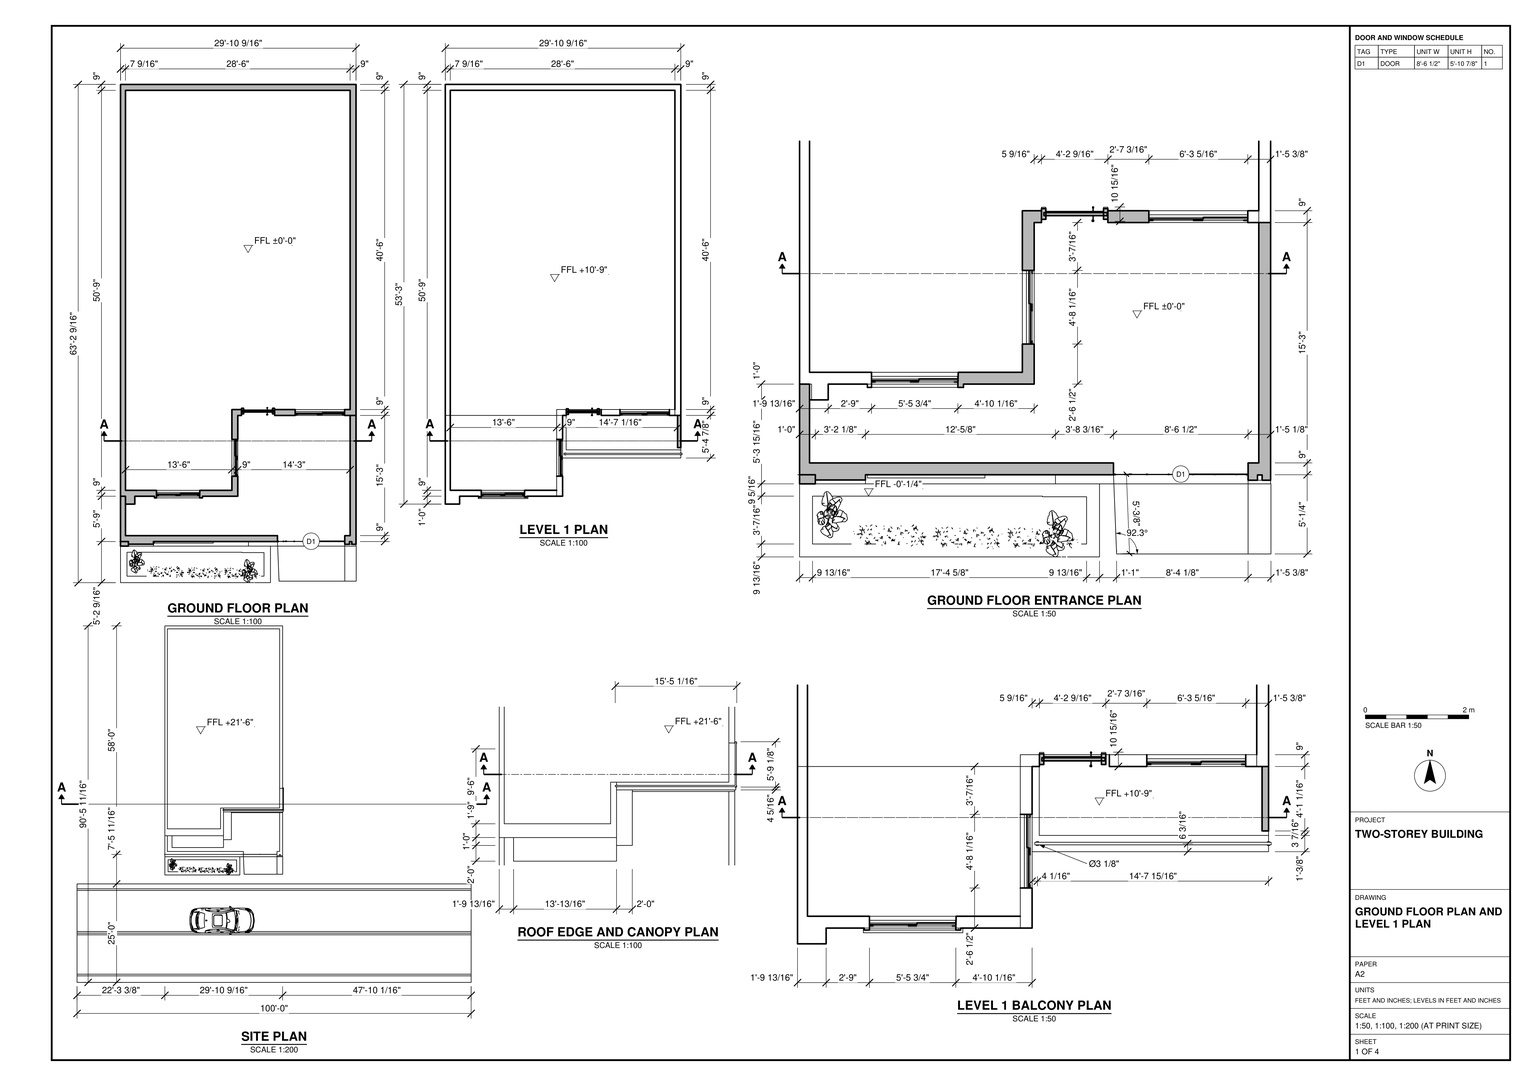
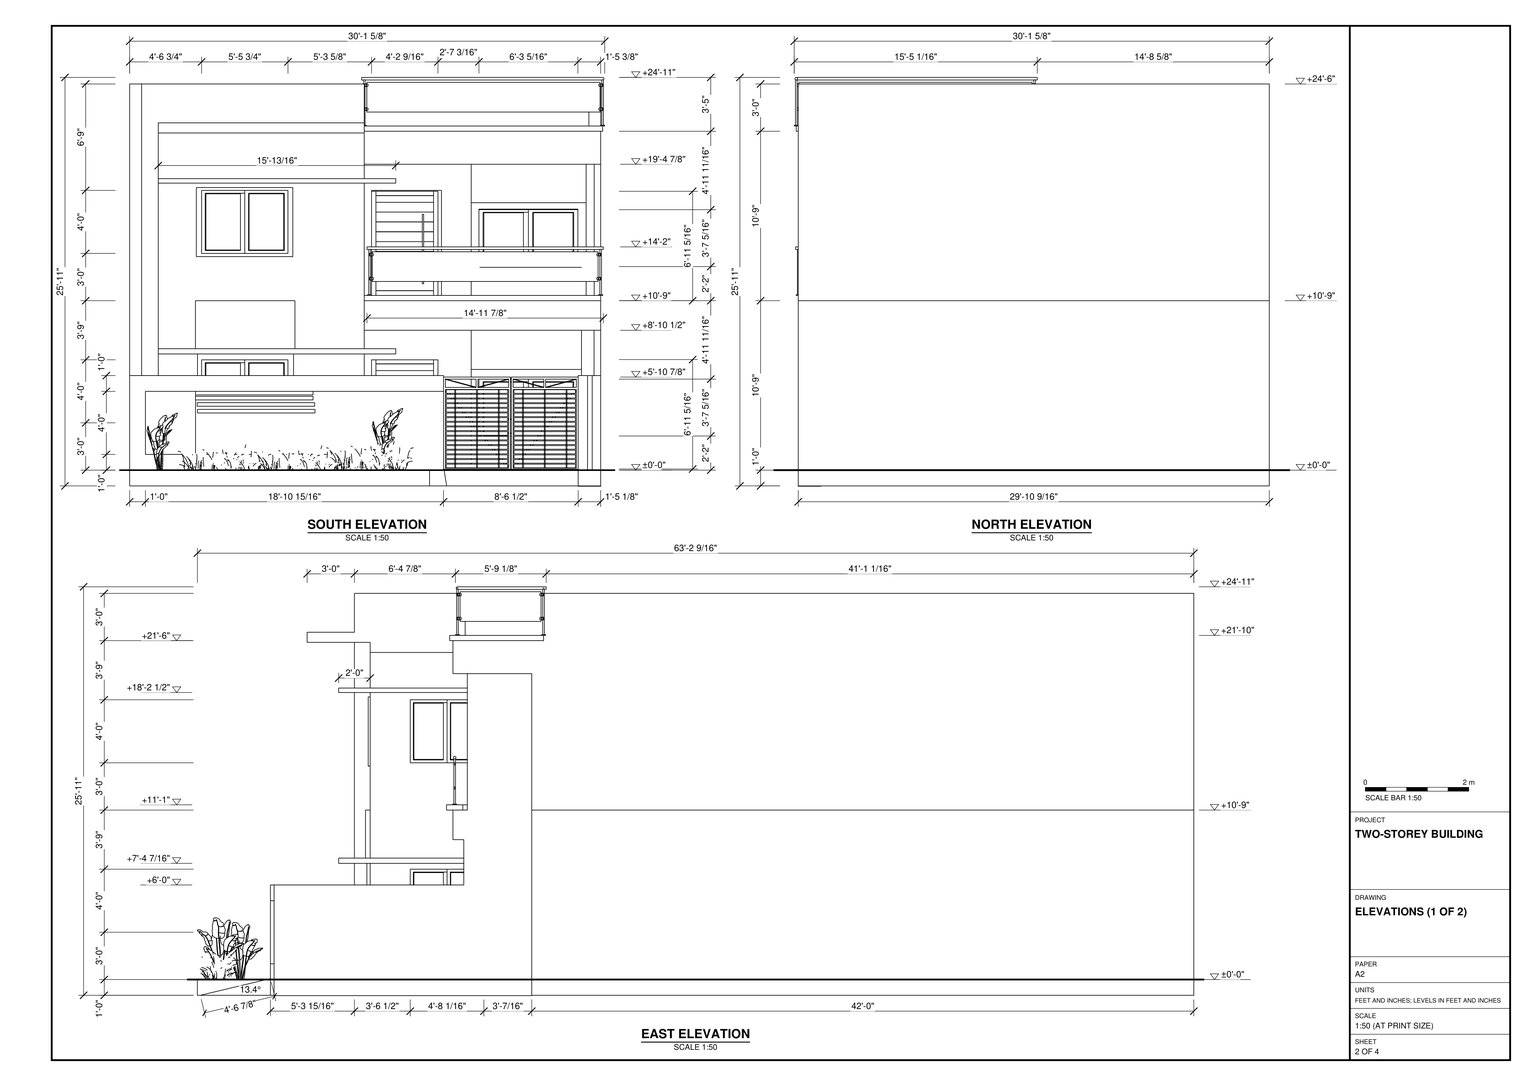
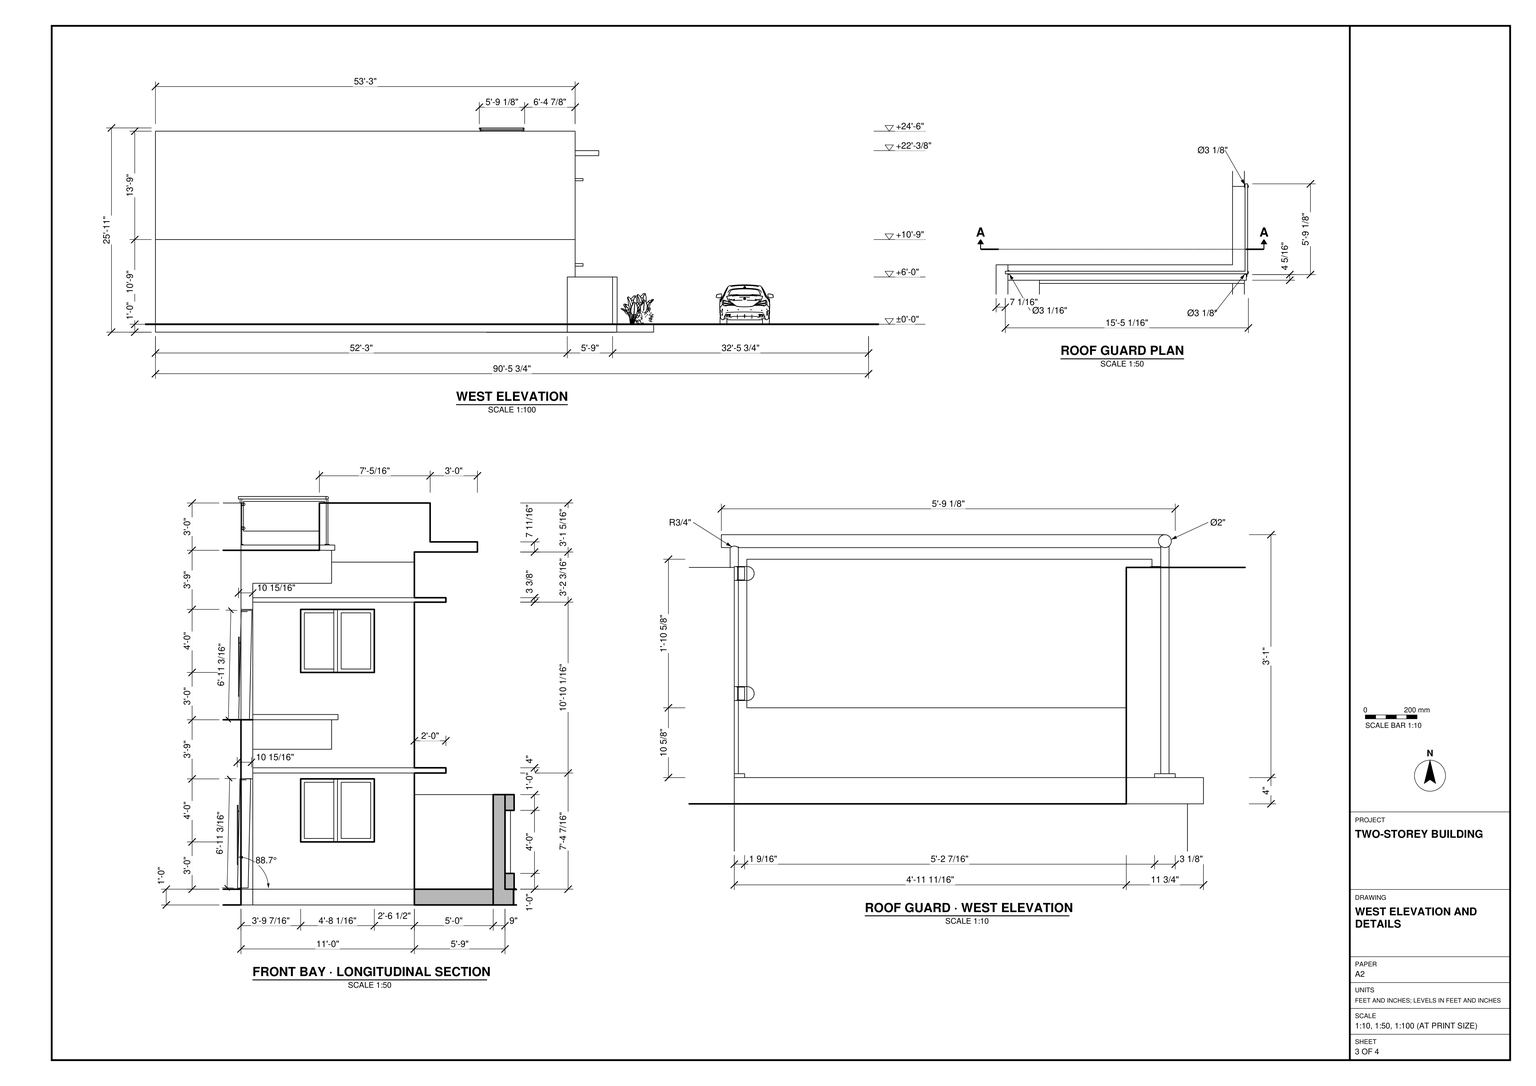
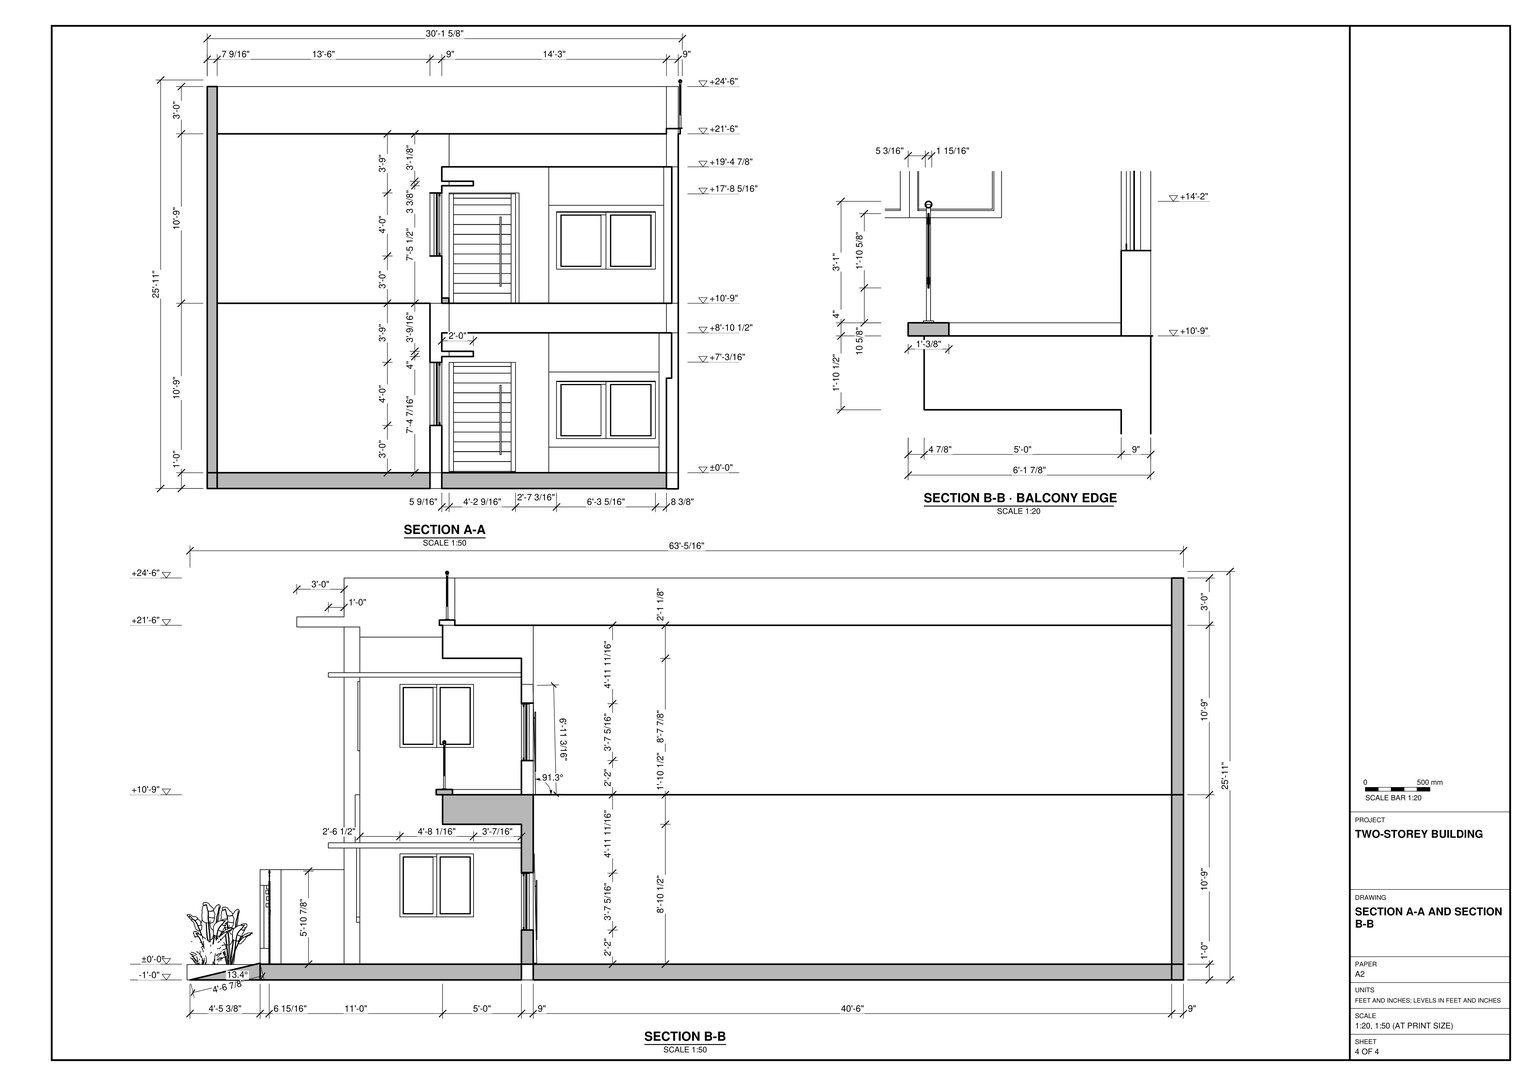
Build the two-storey building and its street frontage in SketchUp from task_files/diagram_01.pdf. Work in feet and inches. Including the site, the model shall measure 100'-0" along X, 90'-5 11/16" along Y and 25'-11 1/4" along Z. Set the ground floor at ±0'-0" and the upper floor at +10'-9".

Use the floor plans to lay out the long side walls, straight rear wall and stepped south wall. Follow the wall thicknesses shown, including the 7 9/16" west wall and 9" east wall of the main block. Model the floor slabs, flat roof and parapets. At the front, use the entrance and balcony plans to place the doors and windows on the correct faces of the stepped wall. Match the projecting canopies at both storeys and the balcony slab and guard on the recessed side. Use the roof guard detail for the posts, panels and top rail where the guard turns the roof corner.

Include the front boundary wall, slatted double gate and planting bed. Place the street across the frontage with the car positioned as in the site plan. Decor and loose items, including the plants and car, may be any suitable library components. Keep shell elements such as walls, slabs and roof, and each furniture or joinery piece, in separate groups or components; use components for repeated parts. Save one SketchUp model as output_files/two_storey_building_stepped_frontage_and_street.skp.

# SketchUp Ruby script. Lengths in inches.
U = 1.inch
M = Sketchup.active_model
def pt(a) = Geom::Point3d.new(a.map { |v| v * U })
def face(e, loops, mat)
  f = e.add_face(loops[0].map { |a| pt(a) })
  loops[1..].each { |l| e.add_face(l.map { |a| pt(a) }).erase! }
  f.material = f.back_material = mat if mat
  f
end
# faces: each face lists its corners as indices into pts; further lists are holes
def faces(e, pts, list, mat = nil) = list.each { |f| face(e, (f[0].is_a?(Array) ? f : [f]).map { |l| l.map { |i| pts[i] } }, mat) }
# xy, xz, yz: faces in a plane at the given z, y or x. An outline is a flat list of corners, or four numbers for a rectangle; further outlines are holes
def ring(l) = l.size == 4 ? [[l[0], l[1]], [l[2], l[1]], [l[2], l[3]], [l[0], l[3]]] : l.each_slice(2).to_a
def flat(e, list, mat, &to3) = list.each { |f| face(e, (f[0].is_a?(Array) ? f : [f]).map { |l| ring(l).map { |u, v| to3.(u, v) } }, mat) }
def xy(e, z, list, mat = nil) = flat(e, list, mat) { |x, y| [x, y, z] }
def xz(e, y, list, mat = nil) = flat(e, list, mat) { |x, z| [x, y, z] }
def yz(e, x, list, mat = nil) = flat(e, list, mat) { |y, z| [x, y, z] }
def lines(e, pts, list) = list.each { |a, b| e.add_line(pt(pts[a]), pt(pts[b])) }
# prism: a flat outline (further loops are holes) pulled along v
def prism(e, loops, v, mat = nil)
  f = face(e, loops, mat); d = Geom::Vector3d.new(v.map { |x| x * U })
  f.pushpull(f.normal.samedirection?(d) ? d.length : -d.length)
end
def box(e, o, s, mat = nil) = prism(e, [[o, [o[0] + s[0], o[1], o[2]], [o[0] + s[0], o[1] + s[1], o[2]], [o[0], o[1] + s[1], o[2]]]], [0, 0, s[2]], mat)
def at(x, y, z, deg = 0) = Geom::Transformation.translation(pt([x, y, z])) * Geom::Transformation.rotation(ORIGIN, Z_AXIS, deg.degrees)
def axes(o, x, y, z) = Geom::Transformation.new([*x, 0, *y, 0, *z, 0, *pt(o).to_a, 1])
def part(name) = M.definitions.add(name)
# library, detail: a bought-in or finely detailed component or shape, given as its bounding box
def library(name, o, s) = part(name).tap { |d| box(d.entities, o, s) }
def detail(e, o, s) = box(e.add_group.entities, o, s)
def put(e, d, t, mat = nil) = e.add_instance(d, t).tap { |i| i.material = mat if mat }
def group(e, t, mat = nil) = e.add_group.tap { |g| g.transformation = t; g.material = mat if mat }.entities
root = M.entities
M.materials.add("[Asphalt_New]").color = [67, 60, 62]
M.materials.add("[Color M00]").color = [255, 255, 255]
M.materials.add("[Granite Dark Gray]").color = [69, 68, 68]
M.materials.add("[Metal Seamed]").color = [118, 119, 115]
M.materials.add("[Stone Brushed Khaki]").color = [226, 197, 133]
M.materials.add("[Stone Vein Gray]").color = [166, 165, 165]
M.materials.add("[Translucent Glass Blue]").color = [100, 149, 237]
M.materials["[Translucent Glass Blue]"].alpha = 0.5
M.materials.add("[Wood Cherry Original]").color = [68, 39, 18]
M.materials.add("[Wood Cherry Original]1").color = [152, 86, 42]
M.materials.add("[Wood Floor Light]").color = [140, 99, 62]
M.materials.add("white").color = [255, 255, 255]
c1 = part("Janela aluminio")
xy(c1.entities,0,[[0,0,47.24,1.57],[23.62,1.57,47.24,2.76],[0,2.76,25.98,3.9375],[0,3.9375,47.24,5.91]])
xy(c1.entities,43.31,[[0,0,47.24,1.57],[23.62,1.57,47.24,2.76],[0,2.76,0,5.91,47.24,5.91,47.24,3.9375,25.98,3.9375,25.98,2.76],[25.98,2.76,47.24,3.9375]])
xz(c1.entities,1.57,[[0,0,23.62,0,23.62,41.34,21.26,41.34,21.26,1.97,1.97,1.97,1.97,41.34,23.62,41.34,23.62,43.31,0,43.31],[[23.62,0,47.24,43.31],[25.7,1.97,45.28,41.34]]])
xz(c1.entities,2.76,[[[0,0,23.62,43.31],[2.36,2.36,21.26,40.94]],[23.62,0,25.98,43.31]])
xz(c1.entities,2.76,[[2.36,2.36,21.26,40.94]],"[Translucent Glass Blue]")
xz(c1.entities,3.9375,[[25.98,0,25.98,2.36,44.88,2.36,44.88,40.94,25.98,40.94,25.98,43.31,47.24,43.31,47.24,0]])
xz(c1.entities,3.9375,[[25.98,2.36,44.88,40.94]],"[Translucent Glass Blue]")
yz(c1.entities,0,[[0,0,1.57,43.31],[2.76,0,5.91,43.31]])
yz(c1.entities,23.62,[[1.57,0,2.76,43.31]])
yz(c1.entities,25.98,[[2.76,0,3.9375,43.31]])
yz(c1.entities,47.24,[[0,0,1.57,43.31],[1.57,0,2.76,43.31],[3.9375,0,5.91,43.31]])
c2 = part("Agrupar\#4")
xy(c2.entities,0,[[0,0,60.82,4.875]],"[Wood Floor Light]")
c3 = part("Agrupar\#7")
box(c3.entities,[0,0,0.25],[0.65,5.875,0.35])
c4 = part("Agrupar\#15")
prism(c4.entities,[[[0,0.625,0],[0.65,0.625,0],[0.65,0,0],[0,0,0]]],[0,0.02,45.16])
c5 = part("Agrupar\#14")
put(c5.entities,c3,at(0,0.65,6.88))
put(c5.entities,c4,at(0,0,0))
put(c5.entities,c3,at(0,0.65,40.25))
c6 = part("Agrupar\#6")
prism(c6.entities,[[[-0.5,0.62,-4.9375],[0.77,0.62,-4.9375],[0.77,-0.19,-4.9375],[-0.5,-0.19,-4.9375]]],[0,0.03,52.91])
c7 = part("Agrupar\#8")
put(c7.entities,c3,at(0,0.65,6.88))
put(c7.entities,c6,at(0,0,0))
put(c7.entities,c3,at(0,0.65,40.25))
c8 = part("Agrupar\#2")
prism(c8.entities,[[[0,2.67,0.04],[55.46,2.67,0.04],[55.46,0.04,0],[0,0.04,0]]],[0,-0.04,3.23],"[Wood Cherry Original]")
c9 = part("Agrupar\#10")
prism(c9.entities,[[[0,3.76,0.04],[4.23,3.76,0.04],[4.23,1.14,0],[0,1.14,0]]],[0,-1.14,83.14],"[Wood Cherry Original]")
c10 = part("Agrupar\#1")
prism(c10.entities,[[[0,3.76,0.04],[4.23,3.76,0.04],[4.23,1.14,0],[0,1.14,0]]],[0,-1.14,83.14],"[Wood Cherry Original]")
c11 = part("Agrupar\#3")
put(c11.entities,c8,at(4.23,0,79.91))
put(c11.entities,c9,at(59.6875,0,0))
put(c11.entities,c10,at(0,0,0))
c12 = part("Agrupar\#5")
put(c12.entities,c11,axes([0,-1.34,0.11],[1,0,0],[0,3.10443,-0.05961],[0,0.0192,0.99982]))
c13 = part("Agrupar\#9")
put(c13.entities,c5,axes([49.36,10.72,17.77],[1,0,0],[0,-1,0],[0,0,1]))
put(c13.entities,c7,at(49.36,0,17.76))
put(c13.entities,c12,at(0,0.21,0.01))
c14 = part("Agrupar\#11")
box(c14.entities,[0,0,0],[60.82,4.875,7.44],"[Wood Floor Light]")
c15 = part("Agrupar\#12")
put(c15.entities,c14,at(0,0,67.34))
put(c15.entities,c14,at(0,0,44.83))
put(c15.entities,c14,at(0,0,59.9))
put(c15.entities,c14,at(0,0,74.78))
put(c15.entities,c14,at(0,0,52.37))
put(c15.entities,c14,at(0,0,7.53))
put(c15.entities,c14,at(0,0,0))
put(c15.entities,c14,at(0,0,29.95))
put(c15.entities,c14,at(0,0,15.07))
put(c15.entities,c14,at(0,0,22.51))
put(c15.entities,c14,at(0,0,37.39))
c16 = part("Agrupar\#13")
put(c16.entities,c13,at(0,0,0.0625))
put(c16.entities,c15,axes([2.375,5.17,0.15],[1,0,0],[0,0.48232,0.01095],[0,-0.02269,0.99974]))
c17 = part("PORTA PIVOTANDE ENVERNIZADA LUXURY")
p = [[59.6875,-1.28,79.91],[59.6875,-3.1,79.89],[4.23,-1.28,79.91],[4.23,-3.1,79.89]]
lines(c17.entities,p,[[0,1],[2,3]])
put(c17.entities,c2,at(0.13,-2.89,82.23))
put(c17.entities,c16,at(0,-6.8,-0.11))
c18 = library("Merbau Gate Metal Frame",[0,0,0],[4.48,115.59,70.87])
c19 = library("Banana Leaf Plant",[-4.48,-0.74,0.58],[37.34,48.6,74.1])
c20 = part("Untitled")
xy(c20.entities,0,[[140,0,145,1200],[150,0,155,1200]])
xy(c20.entities,0,[[0,0,15,1200],[20,0,140,1200],[145,0,150,1200],[155,0,275,1200],[280,0,300,1200]],"[Asphalt_New]")
xy(c20.entities,0,[[15,0,20,1200],[275,0,280,1200]],"white")
c21 = library("mercy",[0,0.0625,0.17],[86.93,197.26,61.05])
c22 = library("Group\#2",[0,0,0],[179.875,3.15,36.98])
c23 = library("Group\#3",[0,0,0],[185.04,69.11,36.98])
c24 = library("Group16",[-203.48,36.63,23.35],[29.68,67.31,27.29])
xy(root,-12.25,[[608.82,385.54,608.82,398.71,616.96,398.71,616.96,581.71,625.96,581.71,625.96,385.54]])
xy(root,-12,[[[267.38,327.15,267.38,383.28,462.18,383.28,462.18,382.78,495.69,382.78,495.69,327.15],[277.22,336.99,485.86,336.99,485.86,372.9375,452.34,372.9375,452.34,373.4375,277.22,373.4375]],[508.72,329.4,506.62,382.78,508.72,382.78],[508.72,329.4,608.82,382.78],[277.22,336.99,277.22,373.4375,452.34,373.4375,452.34,372.9375,485.86,372.9375,485.86,336.99],[506.62,382.78,506.34,389.71,506.34,398.71,274.96,398.71,274.96,458.71,276.5,458.71,276.5,446.71,289.17,446.71,289.17,458.71,445.96,458.71,445.96,581.71,451.52,581.71,451.52,590.71,436.96,590.71,436.96,467.71,274.96,467.71,274.96,1076.71,616.96,1076.71,616.96,590.71,502.08,590.71,502.08,581.71,616.96,581.71,616.96,398.71,608.82,398.71,608.82,382.78],
  [462.18,382.78,495.69,383.28],[495.69,382.78,495.69,383.28,462.18,383.28,462.18,389.71,506.34,389.71,506.62,382.78],[608.82,382.78,625.96,385.54],[267.38,383.28,267.38,458.71,274.96,458.71,274.96,398.71,506.34,398.71,506.34,389.71,462.18,389.71,462.18,383.28],[276.5,446.71,276.5,458.71,267.38,458.71,267.38,1085.71,625.96,1085.71,625.96,581.71,616.96,581.71,616.96,1076.71,274.96,1076.71,274.96,467.71,436.96,467.71,436.96,458.71,289.17,458.71,289.17,446.71]])
xy(root,-0.25,[[[267.38,327.15,495.69,327.15,495.69,382.78,462.18,382.78,462.18,383.28,267.38,383.28],[277.22,336.99,277.22,373.4375,452.34,373.4375,452.34,372.9375,485.86,372.9375,485.86,336.99]]])
xy(root,0,[[267.38,382.78,462.18,383.28],[506.62,382.78,608.82,382.78,608.82,398.71,616.96,398.71,616.96,581.71,502.08,581.71,502.08,590.71,616.96,590.71,616.96,1076.71,274.96,1076.71,274.96,467.71,436.96,467.71,436.96,590.71,451.52,590.71,451.52,581.71,445.96,581.71,445.96,458.71,289.17,458.71,289.17,446.71,274.96,446.71,274.96,398.71,506.34,398.71,506.34,389.71],[462.18,382.78,506.62,382.78,506.34,389.71,462.18,389.71],[608.82,382.78,625.96,385.54],[267.38,383.28,462.18,389.71],
  [615.96,385.54,619.5,389.54],[276.5,446.71,289.17,446.71,289.17,458.71,436.96,458.71,436.96,467.71,274.96,467.71,274.96,1076.71,616.96,1076.71,616.96,581.71,625.96,581.71,625.96,1085.71,267.38,1085.71,267.38,458.71,276.5,458.71],[274.96,446.71,276.5,458.71],[502.08,581.71,616.96,590.71]])
xy(root,12,[[279.38,382.78,317.53,385.71],[317.53,382.78,462.18,389.71],[279.38,385.71,317.53,389.71]])
xy(root,25.99,[[533.27,581.71,608.58,590.71]])
xy(root,31.89,[[319.02,456.21,392.14,458.71]])
xy(root,36,[[322.14,456.21,387.89,456.21,387.89,458.71,388.14,467.71,322.14,467.71],[436.96,489.21,445.96,545.28]])
xy(root,43.52,[[319.03,387.28,408.47,389.71],[319.03,389.71,408.47,391.71]])
xy(root,46.25,[[319.03,387.28,408.47,389.71]])
xy(root,48.65,[[318.8,387.71,408.24,389.71],[318.8,389.71,408.24,391.71]])
xy(root,51.38,[[318.8,387.71,408.24,389.71]])
xy(root,53.47,[[317.53,387.11,406.97,389.11]])
xy(root,57.27,[[317.53,387.71,406.97,389.71]])
xy(root,60,[[279.38,382.78,317.53,385.71],[317.53,382.78,317.53,387.71,406.97,387.71,406.97,389.71,494.34,389.71,494.34,382.78],[494.34,382.78,506.34,389.71],[279.38,385.71,317.53,389.71],[317.53,387.71,406.97,389.71]])
xy(root,69.74,[[533.27,581.71,608.58,590.71]])
xy(root,72,[[267.38,382.78,506.34,389.71],[608.82,385.54,615.96,385.54,615.96,389.54,619.5,389.54,619.5,385.54,625.96,385.54,625.96,529.96,620.89,529.96,620.89,581.71,616.96,581.71,616.96,398.71,608.82,398.71],[267.38,389.71,506.34,389.71,506.34,398.71,274.96,398.71,274.96,446.71,267.38,446.71],[267.38,446.71,274.96,458.71]])
xy(root,84,[[322.14,456.21,322.14,467.71,388.14,467.71,387.89,458.71,387.89,456.21],[387.89,458.71,388.14,467.71,388.14,458.71],[436.96,489.21,445.96,545.28],[451.52,581.71,502.08,590.71]])
xy(root,88.45,[[289.17,434.71,289.17,458.71,319.02,458.71,319.02,456.21,392.14,456.21,392.14,458.71,445.96,458.71,445.96,581.71,469.96,581.71,469.96,434.71],[322.14,456.21,388.14,458.71]])
xy(root,92.4375,[[289.17,434.71,469.96,434.71,469.96,581.71,445.96,581.71,445.96,458.71,393.21,458.71,393.21,455.15,317.46,455.15,317.46,458.71,289.17,458.71],[317.46,455.15,393.21,458.71]])
xy(root,106.5,[[620.89,521.71,625.96,529.96]])
xy(root,106.5,[[445.96,521.71,620.89,581.71]],"[Metal Seamed]")
xy(root,129,[[317.46,455.15,393.21,458.71],[274.96,467.71,436.96,581.71],[445.96,516.84,625.96,521.71],[445.96,521.71,625.96,521.71,625.96,529.24,451.375,529.24,451.375,581.71,445.96,581.71],[451.375,529.24,625.96,529.24,625.96,532.65,621.02,532.65,621.02,581.71,504.76,581.71,504.76,590.71,451.52,590.71,451.52,581.71,451.375,581.71],
  [267.38,581.71,274.96,581.71,274.96,1076.71,616.96,1076.71,616.96,581.71,625.96,581.71,625.96,1085.71,267.38,1085.71],[274.96,581.71,436.96,581.71,436.96,590.71,616.96,590.71,616.96,1076.71,274.96,1076.71],[436.96,581.71,451.52,590.71],[504.76,581.71,616.96,590.71]])
xy(root,133,[[445.96,516.84,625.96,516.84,625.96,529.24,451.375,529.24,451.375,581.71,445.96,581.71]])
xy(root,154.99,[[533.27,581.71,608.58,590.71]])
xy(root,162.5625,[[318.14,457.21,322.14,458.71],[322.14,457.21,390.14,458.71]])
xy(root,165,[[322.14,457.21,387.89,457.21,387.89,458.71,388.14,467.71,322.14,467.71],[436.96,489.21,445.96,545.28]])
xy(root,198.74,[[533.27,581.71,608.58,590.71]])
xy(root,213,[[322.14,457.21,322.14,467.71,388.14,467.71,387.89,458.71,387.89,457.21],[387.89,458.71,388.14,467.71,388.14,458.71],[436.96,489.21,445.96,545.28],[451.52,581.71,504.76,590.71]])
xy(root,215.15,[[318.14,457.21,322.14,458.71],[322.14,457.21,387.58,458.71],[387.58,457.21,390.14,458.71],[390.14,457.21,391.58,458.71]])
xy(root,218.51,[[289.17,434.71,289.17,458.71,445.96,458.71,445.96,581.71,469.96,581.71,469.96,434.71]])
xy(root,232.875,[[445.96,521.71,445.96,581.71,621.02,581.71,621.02,532.65,625.96,532.65,625.96,521.71]],"[Metal Seamed]")
xy(root,256.7,[[289.17,410.71,445.96,458.71]])
xy(root,258,[[274.96,467.71,436.96,467.71,436.96,531.03,616.96,531.03,616.96,1076.71,274.96,1076.71],[445.96,519.28,627.46,521.71],[625.96,521.71,627.46,590.71]])
xy(root,262,[[445.96,519.28,627.46,519.28,627.46,590.71,616.96,590.71,616.96,531.03,445.96,531.03]])
xy(root,264.4,[[289.17,410.71,445.96,446.71]])
xy(root,294,[[267.38,446.71,445.96,446.71,445.96,531.03,436.96,531.03,436.96,467.71,274.96,467.71,274.96,1076.71,616.96,1076.71,616.96,590.71,625.96,590.71,625.96,1085.71,267.38,1085.71]])
xz(root,327.15,[[267.38,-12,495.69,-0.25]])
xz(root,336.99,[[277.22,-12,485.86,-0.25]])
xz(root,372.9375,[[452.34,-12,485.86,-0.25]])
xz(root,373.4375,[[277.22,-12,452.34,-0.25]])
xz(root,382.78,[[462.18,-12,495.69,-0.25],[495.69,-12,625.96,-12,625.96,0,462.18,0,462.18,-0.25,495.69,-0.25],[506.62,0,608.82,0.75]])
xz(root,382.78,[[267.38,0,462.18,0,462.18,12,279.38,12,279.38,60,506.34,60,506.34,72,267.38,72]],"[Metal Seamed]")
xz(root,383.28,[[267.38,-12,462.18,-0.25],[267.38,-0.25,462.18,0]])
xz(root,385.54,[[608.82,-12.25,625.96,-12],[608.82,-12,625.96,0]])
xz(root,385.54,[[608.82,0,615.96,72],[619.5,0,625.96,72]],"[Stone Vein Gray]")
xz(root,385.71,[[279.38,12,317.53,60]],"[Wood Cherry Original]1")
xz(root,387.11,[[317.53,53.47,406.97,56.2]])
xz(root,387.28,[[319.03,43.52,408.47,46.25]])
xz(root,387.71,[[318.8,48.65,408.24,51.38],[317.53,57.27,406.97,60]])
xz(root,389.54,[[615.96,0,619.5,72]],"[Stone Brushed Khaki]")
xz(root,389.71,[[267.38,0,267.38,72,506.34,72,506.34,60,279.38,60,279.38,12,462.18,12,462.18,0]])
xz(root,389.71,[[462.18,-12,506.34,0],[[462.18,0,506.34,0,506.34,60,406.97,60,406.97,57.27,317.53,57.27,317.53,12,462.18,12],[319.03,43.52,408.47,46.25],[318.8,48.65,408.24,51.38]]],"[Stone Brushed Khaki]")
xz(root,398.71,[[608.82,-12.25,616.96,-12],[274.96,-12,506.34,0],[608.82,-12,616.96,0],[274.96,0,506.34,72],[608.82,0,616.96,72]])
xz(root,410.71,[[289.17,256.7,445.96,264.4]])
xz(root,434.71,[[289.17,88.45,469.96,92.4375]])
xz(root,446.71,[[276.5,-12,289.17,0]])
xz(root,446.71,[[276.5,0,289.17,0,289.17,264.4,445.96,264.4,445.96,294,276.5,294]],"[Metal Seamed]")
xz(root,446.71,[[274.96,0,276.5,0,276.5,294,267.38,294,267.38,72,274.96,72]],"[Stone Brushed Khaki]")
xz(root,455.15,[[317.46,92.4375,393.21,129]],"[Wood Cherry Original]1")
xz(root,456.21,[[[319.02,31.89,392.14,88.45],[322.14,36,387.89,84]]],"[Wood Cherry Original]1")
xz(root,457.21,[[[391.58,162.46,391.58,215.15,318.14,215.15,318.14,162.5625,390.14,162.5625],[322.14,165,387.89,213]]],"[Granite Dark Gray]")
xz(root,458.71,[[267.38,-12,274.96,0],[274.96,-12,276.5,0],[289.17,-12,436.96,0],[267.38,0,274.96,72],[322.14,88.45,388.14,92.4375]])
xz(root,458.71,[[436.96,-12,445.96,0],[289.17,0,445.96,0,445.96,88.45,392.14,88.45,392.14,31.89,319.02,31.89,319.02,88.45,289.17,88.45],[[289.17,92.4375,317.46,92.4375,317.46,129,393.21,129,393.21,92.4375,445.96,92.4375,445.96,218.51,289.17,218.51],[391.58,162.46,390.14,162.5625,318.14,162.5625,318.14,215.15,391.58,215.15]],[289.17,221.91,445.96,256.7]],"[Stone Brushed Khaki]")
xz(root,467.71,[[274.96,-12,436.96,0],[274.96,0,274.96,129,388.14,129,388.14,84,322.14,84,322.14,36,388.14,36,388.14,129,436.96,129,436.96,0],[274.96,129,274.96,258,388.14,258,388.14,213,322.14,213,322.14,165,388.14,165,388.14,258,436.96,258,436.96,129],[274.96,258,436.96,294]])
xz(root,489.21,[[436.96,36,445.96,84],[436.96,165,445.96,213]])
xz(root,516.84,[[445.96,129,625.96,133]])
xz(root,519.28,[[445.96,258,627.46,262]])
xz(root,521.71,[[445.96,106.5,625.96,129],[445.96,232.875,625.96,258]],"[Metal Seamed]")
xz(root,529.24,[[451.375,129,625.96,133]])
xz(root,529.96,[[620.89,72,625.96,106.5]],"[Stone Brushed Khaki]")
xz(root,531.03,[[436.96,258,445.96,294],[445.96,258,616.96,262]])
xz(root,532.65,[[621.02,129,625.96,232.875]],"[Stone Brushed Khaki]")
xz(root,545.28,[[436.96,36,445.96,84],[436.96,165,445.96,213]])
xz(root,581.71,[[616.96,-12.25,625.96,-12],[502.08,-12,527.38,0],[527.38,-12,611.35,0],[611.35,-12,616.96,0],[616.96,-12,625.96,0],
  [611.35,0,616.96,0,616.96,72,620.89,72,620.89,106.5,611.35,106.5],[616.96,0,616.96,72,620.89,72,620.89,106.5,625.96,106.5,625.96,0],[445.96,129,451.375,133],[614.9,129,621.02,232.875],[621.02,129,625.96,232.875]])
xz(root,581.71,[[445.96,-12,451.52,-12,451.52,84,502.08,84,502.08,0,527.38,0,527.38,106.5,445.96,106.5,445.96,92.4375,469.96,92.4375,469.96,88.45,445.96,88.45],[451.375,129,451.52,129,451.52,213,504.76,213,504.76,129,527.38,129,527.38,232.875,445.96,232.875,445.96,221.91,469.96,221.91,469.96,218.51,445.96,218.51,445.96,133,451.375,133]],"[Stone Brushed Khaki]")
xz(root,581.71,[[527.38,0,611.35,19.48],[[527.38,19.48,611.35,76.6875],[533.27,25.99,608.58,69.74]],[527.38,76.6875,611.35,106.5],[[527.38,129,614.9,203.59],[533.27,154.99,608.58,198.74]],[527.38,203.59,614.9,232.875]],"[Wood Cherry Original]1")
xz(root,590.71,[[436.96,-12,451.52,129],[502.08,-12,616.96,0],[[502.08,0,502.08,84,451.52,84,451.52,129,616.96,129,616.96,0],[533.27,25.99,608.58,69.74]],[625.96,258,627.46,262],[616.96,262,625.96,294]])
xz(root,1076.71,[[274.96,-12,616.96,0],[274.96,0,616.96,129],[274.96,129,616.96,258],[274.96,258,616.96,294]])
xz(root,1085.71,[[267.38,-12,625.96,129],[267.38,129,625.96,294]])
yz(root,267.38,[[327.15,-12,383.28,-0.25],[383.28,-12,383.28,0,389.71,0,389.71,72,458.71,72,458.71,-12],[458.71,-12,1085.71,0],[382.78,0,389.71,72],[458.71,0,1085.71,0,1085.71,129,446.71,129,446.71,72,458.71,72],
  [446.71,129,1085.71,294]])
yz(root,274.96,[[398.71,-12,458.71,0],[467.71,-12,1076.71,0],[398.71,0,446.71,72],[446.71,0,458.71,72],[467.71,0,1076.71,129],
  [467.71,129,1076.71,258],[467.71,258,1076.71,294]])
yz(root,276.5,[[446.71,-12,458.71,0]])
yz(root,277.22,[[336.99,-12,373.4375,-0.25]])
yz(root,279.38,[[382.78,12,385.71,60],[385.71,12,389.71,60]])
yz(root,289.17,[[446.71,-12,458.71,0],[446.71,0,458.71,88.45],[434.71,88.45,446.71,92.4375],[446.71,92.4375,458.71,218.51],[434.71,218.51,446.71,221.91],
  [446.71,221.91,458.71,256.7],[410.71,256.7,446.71,264.4]])
yz(root,317.46,[[455.15,92.4375,458.71,129]])
yz(root,317.53,[[385.71,12,389.71,12,389.71,57.27,387.71,57.27,387.71,60,385.71,60]])
yz(root,318.14,[[457.21,162.5625,458.71,215.15]])
yz(root,318.8,[[387.71,48.65,389.71,51.38]])
yz(root,319.02,[[456.21,31.89,458.71,87.76],[456.21,87.76,458.71,88.45]])
yz(root,319.03,[[387.28,43.52,389.71,46.25]])
yz(root,322.14,[[456.21,36,467.71,84],[457.21,165,467.71,213]])
yz(root,387.89,[[456.21,36,458.71,84],[457.21,165,458.71,213]])
yz(root,391.58,[[457.21,162.46,458.71,215.15]])
yz(root,392.14,[[456.21,31.89,458.71,35.89],[456.21,35.89,458.71,88.45]])
yz(root,393.21,[[455.15,92.4375,458.71,129]])
yz(root,406.97,[[387.11,53.47,389.11,56.2],[387.71,57.27,389.71,60]])
yz(root,408.24,[[387.71,48.65,389.71,51.38],[389.71,48.65,391.71,51.38]])
yz(root,408.47,[[387.28,43.52,389.71,46.25],[389.71,43.52,391.71,46.25]])
yz(root,436.96,[[458.71,-12,467.71,0],[467.71,-12,590.71,0],[[467.71,0,590.71,129],[489.21,36,545.28,84]],[467.71,258,531.03,294]])
yz(root,445.96,[[516.84,129,581.71,133],[458.71,249,458.71,256.7,410.71,256.7,410.71,264.4,446.71,264.4,446.71,294,531.03,294,531.03,262,519.28,262,519.28,258,521.71,258,521.71,249]])
yz(root,445.96,[[[458.71,-12,581.71,88.45],[489.21,36,545.28,84]],[[458.71,92.4375,458.71,218.51,581.71,218.51,581.71,133,516.84,133,516.84,129,521.71,129,521.71,106.5,581.71,106.5,581.71,92.4375],[489.21,165,545.28,213]],[458.71,221.91,581.71,221.91,581.71,232.875,521.71,232.875,521.71,249,458.71,249]],"[Stone Brushed Khaki]")
yz(root,451.375,[[529.24,129,581.71,133]])
yz(root,451.52,[[581.71,-12,590.71,84],[581.71,129,590.71,213]])
yz(root,452.34,[[372.9375,-12,373.4375,-0.25]])
yz(root,462.18,[[382.78,-12,383.28,-0.25],[383.28,-12,389.71,0],[382.78,-0.25,383.28,0],[382.78,0,389.71,12]])
yz(root,469.96,[[434.71,88.45,581.71,92.4375],[434.71,218.51,581.71,221.91]])
yz(root,485.86,[[336.99,-12,372.9375,-0.25]])
yz(root,495.69,[[327.15,-12,382.78,-0.25]])
yz(root,502.08,[[581.71,-12,590.71,0],[581.71,0,590.71,84]])
yz(root,504.76,[[581.71,129,590.71,213]])
yz(root,506.34,[[389.71,-12,398.71,0],[389.71,0,398.71,72],[382.78,60,389.71,72]])
yz(root,533.27,[[581.71,25.99,590.71,69.74],[581.71,154.99,590.71,198.74]])
yz(root,608.58,[[581.71,25.99,590.71,69.74],[581.71,154.99,590.71,198.74]])
yz(root,608.82,[[385.54,-12.25,398.71,-12],[329.4,-12,382.78,0.75,382.78,0,385.54,0,385.54,-12],[385.54,-12,398.71,0],[385.54,0,398.71,72]])
yz(root,615.96,[[385.54,0,389.54,72]])
yz(root,616.96,[[398.71,-12.25,581.71,-12],[398.71,-12,581.71,0],[581.71,-12,590.71,0],[590.71,-12,1076.71,0],[398.71,0,581.71,72],
  [590.71,0,1076.71,129],[590.71,129,1076.71,258],[531.03,258,590.71,262],[590.71,258,1076.71,294]])
yz(root,619.5,[[385.54,0,389.54,72]])
yz(root,620.89,[[529.96,72,581.71,106.5]])
yz(root,621.02,[[532.65,129,581.71,232.875]])
yz(root,625.96,[[382.78,-12,385.54,0],[516.84,129,529.24,133],[581.71,129,1085.71,129,1085.71,294,590.71,294,590.71,258,521.71,258,521.71,232.875,581.71,232.875]])
yz(root,625.96,[[581.71,0,1085.71,129]],"[Color M00]")
yz(root,625.96,[[385.54,-12.25,581.71,-12.25,581.71,232.875,532.65,232.875,532.65,129,521.71,129,521.71,106.5,529.96,106.5,529.96,72,385.54,72],[581.71,-12,1085.71,0]],"[Stone Brushed Khaki]")
yz(root,627.46,[[519.28,258,590.71,262]])
p = [[506.62,382.78,0],[506.74,379.64,0],[508.72,329.4,-12],[506.62,382.78,-12],[506.34,389.71,-12],[506.34,389.71,0],
  [608.82,382.78,0.75],[506.62,382.78,0.75],[608.82,329.4,-12],[387.89,458.71,36],[387.89,458.71,84],[388.14,467.71,84],
  [388.14,467.71,36],[390.14,458.71,162.5625],[391.58,458.71,162.46],[391.58,457.21,162.46],[390.14,457.21,162.5625],[387.89,458.71,165],
  [387.89,458.71,213],[388.14,467.71,213],[388.14,467.71,165],[265.96,389.71,0],[267.38,389.71,0],[451.52,590.71,213],
  [451.52,590.71,258],[436.96,467.71,129],[436.96,458.71,129],[625.96,590.71,258],[625.96,590.71,257.91],[533.91,522.94,154.4],
  [611.35,522.94,154.4],[626.22,382.78,-12],[626.22,329.4,-12],[625.96,382.78,-12]]
faces(root,p,[[0,1,2,3,4,5],[6,7,1,2,8],[9,10,11,12],[13,14,15,16],[17,18,19,20]])
lines(root,p,[[21,22],[23,24],[25,26],[27,28],[29,30],[31,32],[33,31],[32,8]])
put(root,c1,axes([533.27,581.71,154.99],[1.59411,0,0],[0,1,0],[0,0,1]))
put(root,c1,axes([533.27,581.71,25.99],[1.59411,0,0],[0,1,0],[0,0,1]))
put(root,c1,axes([322.14,458.71,165],[1.39151,0,0],[0,1,0],[0,0,1.10836]))
put(root,c1,axes([322.14,458.71,36],[1.39151,0,0],[0,1,0],[0,0,1.10836]))
put(root,c1,axes([445.96,489.21,165],[0,1.18666,0],[-1,0,0],[0,0,1.10836]))
put(root,c1,axes([445.96,489.21,36],[0,1.18666,0],[-1,0,0],[0,0,1.10836]))
put(root,c17,axes([451.52,589.64,0.99],[0.79102,0,0],[0,1,0],[0,0,0.9999]))
put(root,c17,axes([451.52,588.71,129.11],[0.79102,0,0],[0,1,0],[0,0,0.9999]))
put(root,c18,axes([608.82,389.71,0],[0,0.22806,0],[-0.88649,0,0],[0,0,1]))
put(root,c19,axes([303.83,341.69,-12.44],[-0.75,0,0],[0,0.75,0],[0,0,0.75]))
put(root,c19,axes([475.32,327.15,-8.87],[-0.75,0,0],[0,0.75,0],[0,0,0.75]))
put(root,c20,at(0,300,0,-90))
put(root,c21,at(342.86,231.93,-0.17,-90))
g1 = group(root,at(289.17,434.71,218.51))
xy(g1,3.39,[[0,0,180.79,0,180.79,147,156.79,147,156.79,24,0,24]])
xz(g1,0,[[0,0,180.79,3.39]])
put(root,c22,at(448.05,521.47,133))
put(root,c23,at(443.99,523.58,262))
put(root,c24,at(267.1,154.97,-31.04,-90))
put(root,c24,at(324.91,153.35,-31.74,-90))
put(root,c24,at(380,152.85,-28.42,-90))
